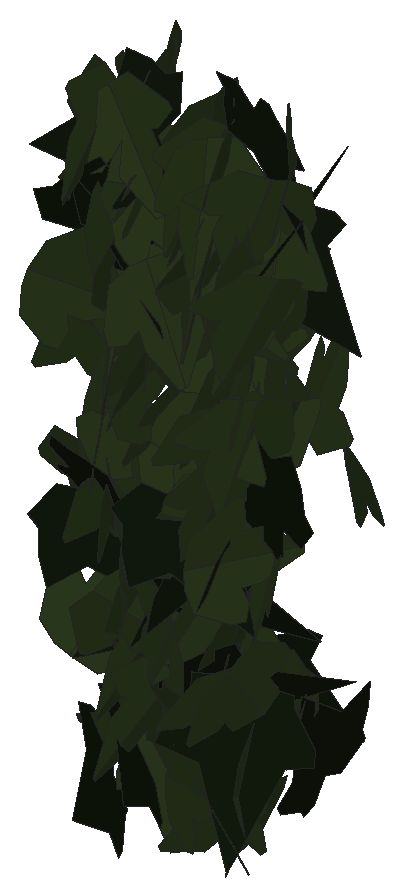
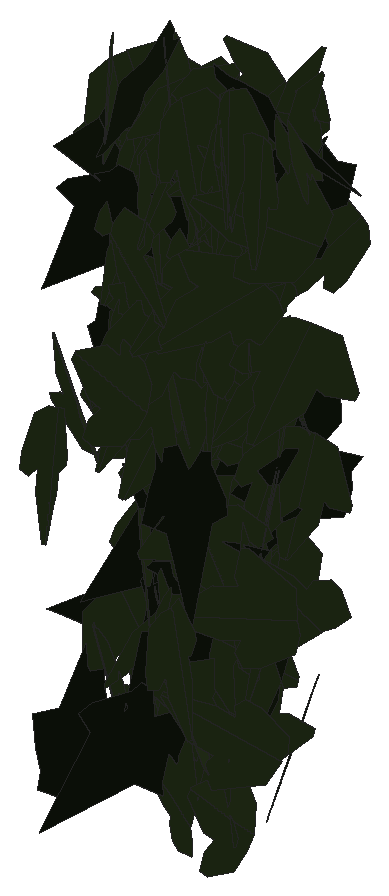
# SketchUp Ruby script. Lengths in inches.
U = 1.inch
M = Sketchup.active_model
def pt(a) = Geom::Point3d.new(a.map { |v| v * U })
def face(e, loops, mat)
  f = e.add_face(loops[0].map { |a| pt(a) })
  loops[1..].each { |l| e.add_face(l.map { |a| pt(a) }).erase! }
  f.material = f.back_material = mat if mat
  f
end
# faces: each face lists its corners as indices into pts; further lists are holes
def faces(e, pts, list, mat = nil) = list.each { |f| face(e, (f[0].is_a?(Array) ? f : [f]).map { |l| l.map { |i| pts[i] } }, mat) }
# xy, xz, yz: faces in a plane at the given z, y or x. An outline is a flat list of corners, or four numbers for a rectangle; further outlines are holes
def ring(l) = l.size == 4 ? [[l[0], l[1]], [l[2], l[1]], [l[2], l[3]], [l[0], l[3]]] : l.each_slice(2).to_a
def flat(e, list, mat, &to3) = list.each { |f| face(e, (f[0].is_a?(Array) ? f : [f]).map { |l| ring(l).map { |u, v| to3.(u, v) } }, mat) }
def xy(e, z, list, mat = nil) = flat(e, list, mat) { |x, y| [x, y, z] }
def xz(e, y, list, mat = nil) = flat(e, list, mat) { |x, z| [x, y, z] }
def yz(e, x, list, mat = nil) = flat(e, list, mat) { |y, z| [x, y, z] }
def lines(e, pts, list) = list.each { |a, b| e.add_line(pt(pts[a]), pt(pts[b])) }
# prism: a flat outline (further loops are holes) pulled along v
def prism(e, loops, v, mat = nil)
  f = face(e, loops, mat); d = Geom::Vector3d.new(v.map { |x| x * U })
  f.pushpull(f.normal.samedirection?(d) ? d.length : -d.length)
end
def box(e, o, s, mat = nil) = prism(e, [[o, [o[0] + s[0], o[1], o[2]], [o[0] + s[0], o[1] + s[1], o[2]], [o[0], o[1] + s[1], o[2]]]], [0, 0, s[2]], mat)
def at(x, y, z, deg = 0) = Geom::Transformation.translation(pt([x, y, z])) * Geom::Transformation.rotation(ORIGIN, Z_AXIS, deg.degrees)
def axes(o, x, y, z) = Geom::Transformation.new([*x, 0, *y, 0, *z, 0, *pt(o).to_a, 1])
def part(name) = M.definitions.add(name)
# library, detail: a bought-in or finely detailed component or shape, given as its bounding box
def library(name, o, s) = part(name).tap { |d| box(d.entities, o, s) }
def detail(e, o, s) = box(e.add_group.entities, o, s)
def put(e, d, t, mat = nil) = e.add_instance(d, t).tap { |i| i.material = mat if mat }
def group(e, t, mat = nil) = e.add_group.tap { |g| g.transformation = t; g.material = mat if mat }.entities
root = M.entities
M.materials.add("efeu1").color = [18, 25, 13]
M.materials.add("efeu2").color = [43, 57, 29]
c1 = part("ivyleaf_10")
p = [[0,0.5,-0.03],[-0.0625,2.02,-0.43],[-0.19,2.01,-0.46],[-0.54,1.05,-0.29],[-0.52,0.625,-0.18],[-0.83,0.76,-0.28],
  [-1.16,0.64,-0.33],[-1.15,0.33,-0.24],[-0.77,-0.39,0.02],[-0.3,-0.51,0.16],[0.04,-0.48,0.23],[-0.02,2.01,-0.4375],
  [-0.06,2.01,-0.43],[0.04,-0.49,0.23],[0.67,-0.49,0.14],[1.38,0.36,-0.2],[1.375,0.51,-0.24],[0.81,0.65,-0.19],
  [0.62,0.59,-0.15],[0.6,1.09,-0.28],[0.5,1.23,-0.31]]
faces(c1.entities,p,[[0,1,2,3,4,5,6,7,8,9,10],[11,12,0,13,14,15,16,17,18,19,20]],"efeu2")
c2 = part("ivyleaf_9")
p = [[1.54,2.16,1.25],[1.36,2.04,1.19],[-0.21,0.99,0.68],[-0.71,1.11,0.82],[-0.85,0.86,0.67],[-0.8,0.17,0.21],
  [-0.9,-0.01,0.1],[-0.67,-0.16,-0.02],[-0.08,-0.08,-0.05],[-0.03,-0.6,-0.4],[0.65,-0.88,-0.66],[0.83,-0.6,-0.49],
  [1.29,-0.42,-0.43],[1.8125,-0.07,-0.26],[1.21,0.44,0.15]]
faces(c2.entities,p,[[0,1,2,3,4,5,6,7,8,9,10,11,12,13,14]],"efeu1")
put(root,c1,axes([20.35,225.55,213.74],[-0.42421,0.23206,0.12727],[-0.13813,0.01099,-0.48042],[-0.22577,-0.44275,0.05478]))
put(root,c1,axes([20.23,225.05,211.57],[-0.33203,-0.30971,-0.20937],[0.1615,0.13372,-0.45391],[0.33715,-0.36905,0.01124]))
put(root,c1,axes([20.32,224.85,210.26],[-0.49854,0.03694,-0.0095],[0.00919,-0.0046,-0.49989],[-0.03702,-0.49861,0.00391]))
put(root,c1,axes([20.1875,225.09,213.93],[0.17199,-0.334,0.32994],[0.20812,-0.26073,-0.37243],[0.42084,0.26545,0.04934]))
put(root,c1,axes([19.99,225.76,209.06],[0.04249,-0.00209,0.49819],[0.40181,0.29574,-0.03303],[-0.29452,0.40316,0.02681]))
put(root,c1,axes([20.03,225.95,207.71],[0.24051,0.01866,-0.43796],[0.42744,0.10078,0.23903],[0.09719,-0.48938,0.03253]))
put(root,c1,axes([20.68,226.42,208.93],[-0.33019,0.13434,0.35061],[-0.33474,0.10614,-0.35592],[-0.17006,-0.46977,0.01985]))
put(root,c1,axes([20.4375,225.74,206.65],[0.14857,-0.34389,0.33116],[-0.11319,0.31157,0.37432],[-0.4638,-0.18619,0.01473]))
put(root,c1,axes([20.18,225.2,212.86],[-0.04588,-0.26731,0.42005],[0.27754,0.33648,0.24444],[-0.41336,0.25559,0.11751]))
put(root,c1,axes([20.53,225.05,208.63],[-0.22189,0.36487,0.26007],[-0.12953,0.22558,-0.42701],[-0.42894,-0.25687,-0.00559]))
put(root,c1,axes([20.53,225.11,211.0625],[-0.0182,0.02508,0.49904],[-0.16563,0.47084,-0.0297],[-0.47142,-0.16639,-0.00883]))
put(root,c1,axes([20.39,224.25,212.4],[0.08449,0.23876,0.43111],[0.03337,0.43362,-0.24669],[-0.49168,0.07045,0.05734]))
put(root,c1,axes([20.34,224.81,208.51],[0.37458,0.16086,-0.28951],[0.24278,0.16391,0.4052],[0.22526,-0.44414,0.04469]))
put(root,c2,axes([20.41,225.08,206.9],[-0.00427,-0.18194,0.4657],[-0.00756,-0.46564,-0.18199],[0.49992,-0.0086,0.00122]))
put(root,c1,axes([20.45,224.9,213.9375],[0.03692,-0.24307,0.43538],[0.20982,-0.38847,-0.23467],[0.45234,0.20003,0.07332]))
put(root,c1,axes([20.62,225.56,214.13],[0.10374,-0.45853,-0.17026],[0.0077,0.17555,-0.4681],[0.48906,0.0945,0.04349]))
put(root,c1,axes([20.6,224.87,210.22],[-0.09866,-0.40844,-0.271],[0.08151,0.25892,-0.4199],[0.48334,-0.12703,0.0155]))
put(root,c2,axes([20.47,224.69,210],[0.05034,-0.28739,-0.40604],[-0.0587,0.40183,-0.29169],[0.49398,0.07703,0.00672]))
put(root,c2,axes([21.04,224.89,213.85],[-0.39263,0.17549,0.25504],[-0.23259,0.10463,-0.43006],[-0.20431,-0.45635,-0.00053]))
put(root,c1,axes([20.55,224.81,211.17],[0.31965,-0.31389,0.22203],[0.16947,-0.14415,-0.44777],[0.34511,0.36152,0.01423]))
put(root,c1,axes([20.8125,225.66,206.73],[0.41253,-0.1131,0.2589],[-0.25032,0.06611,0.42775],[-0.13099,-0.48253,-0.00207]))
put(root,c1,axes([20.72,225.52,214.04],[0.2006,-0.44315,-0.11565],[-0.00035,0.12611,-0.48383],[0.45799,0.1942,0.05028]))
put(root,c1,axes([20.79,225.19,207.3],[-0.49327,-0.06669,-0.04734],[-0.04611,-0.01224,0.49772],[-0.06755,0.49538,0.00593]))
put(root,c2,axes([20.86,225.93,210.35],[0.29065,0.05672,-0.40287],[-0.40003,-0.05043,-0.29569],[-0.07418,0.49421,0.01607]))
put(root,c1,axes([20.78,224.57,210.31],[0.18456,-0.30964,-0.3465],[-0.03849,0.36136,-0.34342],[0.46309,0.15343,0.10955]))
put(root,c1,axes([21.03,224.83,211.83],[-0.38527,-0.00181,0.31869],[-0.31868,0.00717,-0.38522],[-0.00317,-0.49995,-0.00668]))
put(root,c1,axes([20.76,225.41,211.69],[-0.12886,-0.28149,0.39263],[0.08962,-0.41323,-0.26685],[0.47473,0.00161,0.15695]))
put(root,c2,axes([20.4,224.59,210.26],[0.42293,-0.17193,0.2039],[0.18841,-0.07796,-0.45653],[0.18877,0.46299,-0.00116]))
put(root,c1,axes([20.65,225.09,208.6875],[0.31954,-0.37028,-0.10385],[0.06589,-0.08032,0.48909],[-0.37888,-0.32626,-0.00253]))
put(root,c1,axes([20.83,224.77,210.58],[0.02375,0.4817,-0.1319],[-0.00289,0.13218,0.4822],[0.49943,-0.02215,0.00907]))
put(root,c2,axes([20.5,224.84,213.05],[0.28042,-0.40259,0.09636],[0.05111,-0.08182,-0.4906],[0.41079,0.285,-0.00473]))
put(root,c2,axes([20.42,224.65,212.79],[0.1692,0.01649,0.47021],[0.46785,0.04707,-0.17],[-0.04987,0.49751,0.0005]))
put(root,c1,axes([20.52,225.52,212.25],[0.21402,0.18153,0.41381],[0.26213,0.32309,-0.2773],[-0.36808,0.33565,0.04313]))
put(root,c1,axes([20.57,225.1,209.3125],[0.03419,-0.08632,0.4913],[0.37292,-0.32265,-0.08264],[0.3313,0.37209,0.04232]))
put(root,c1,axes([20.79,224.6875,210.25],[-0.20306,-0.37306,-0.2638],[0.14297,0.2223,-0.42443],[0.43396,-0.2478,0.01639]))
put(root,c1,axes([20.86,225.7,209.69],[0.39943,0.2764,-0.11856],[-0.09335,-0.07344,-0.48569],[-0.2859,0.41014,-0.00707]))
put(root,c1,axes([20.76,225.11,208.45],[0.02032,-0.14872,0.47694],[0.20688,-0.43198,-0.14352],[0.45474,0.20317,0.04398]))
put(root,c1,axes([20.82,225.85,207.86],[0.23116,-0.38342,0.22261],[0.09801,-0.20065,-0.44736],[0.43239,0.25046,-0.01761]))
put(root,c1,axes([20.97,224.1875,212.86],[0.0093,0.03412,-0.49875],[-0.05156,0.49624,0.03298],[0.49725,0.05082,0.01275]))
put(root,c2,axes([21.2,225.51,209.125],[-0.43767,-0.17221,0.16968],[-0.1582,-0.06135,-0.47033],[0.18281,-0.46538,-0.00079]))
put(root,c2,axes([20.75,225.03,207.33],[0.01301,-0.23055,0.44348],[0.08072,-0.43684,-0.22947],[0.49327,0.07757,0.02585]))
put(root,c1,axes([20.64,226.25,206.96],[-0.06938,-0.00166,0.49516],[0.47617,-0.13736,0.06626],[0.13581,0.48076,0.02064]))
put(root,c1,axes([20.8125,224.64,209.05],[-0.3066,-0.16633,-0.35823],[0.30662,0.18561,-0.34861],[0.24896,-0.43345,-0.01181]))
put(root,c1,axes([20.91,225.4,207.28],[0.31898,0.38503,-0.00009],[-0.00391,0.00312,-0.49997],[-0.38501,0.31897,0.005]))
put(root,c1,axes([21.03,225.03,208.06],[0.01427,-0.30623,0.39499],[0.03793,-0.39335,-0.30633],[0.49836,0.0387,0.012]))
put(root,c1,axes([20.93,224.88,208.84],[-0.01111,-0.42401,0.26475],[0.04726,0.26274,0.42277],[-0.49764,0.03442,0.03424]))
put(root,c1,axes([21.0625,225.0625,213.43],[0.02805,-0.45958,-0.19494],[0.02291,0.19622,-0.45932],[0.49869,0.01684,0.03206]))
put(root,c1,axes([20.74,224.73,214.05],[0.3627,0.04762,0.34085],[0.3404,0.02337,-0.36549],[-0.05074,0.49718,-0.01547]))
put(root,c1,axes([21.1875,224.33,211.49],[-0.01977,0.04872,0.49723],[-0.19779,0.4562,-0.05256],[-0.45879,-0.19877,0.00124]))
put(root,c1,axes([21.1875,224.57,211.74],[0.10338,-0.43156,-0.23036],[-0.06496,0.22125,-0.44365],[0.48486,0.12165,-0.01032]))
put(root,c1,axes([20.92,224.71,213.4],[-0.05814,-0.19727,-0.45575],[0.32626,0.33077,-0.18479],[0.3744,-0.31887,0.09026]))
put(root,c1,axes([21.16,225.37,209.58],[-0.11444,-0.3912,0.2896],[0.04,-0.30405,-0.39491],[0.48508,-0.06722,0.10088]))
put(root,c1,axes([21.18,225.53,213.85],[-0.01947,-0.49945,-0.01301],[-0.00142,0.01308,-0.49983],[0.49962,-0.01943,-0.00193]))
put(root,c1,axes([21.13,224.99,213.47],[-0.15831,-0.41361,-0.23209],[0.10317,0.20878,-0.44245],[0.46292,-0.18798,0.01924]))
put(root,c1,axes([21.2,224.92,211.17],[-0.01052,-0.43562,-0.2452],[0.00108,0.24523,-0.43573],[0.49989,-0.0097,-0.00422]))
put(root,c1,axes([21.1,225.39,212.14],[-0.0826,-0.21026,-0.44606],[0.16002,0.41637,-0.2259],[0.46644,-0.18008,-0.0015]))
put(root,c1,axes([21.16,224.89,208.9],[-0.27202,0.36763,0.20212],[0.09832,-0.17832,0.45666],[0.40785,0.28818,0.02472]))
put(root,c2,axes([21.15,226.15,207.71],[0.02051,-0.082,-0.4928],[-0.06213,0.48897,-0.08395],[0.4957,0.06468,0.00987]))
put(root,c1,axes([21.27,225.37,213.35],[0.49757,0.04734,-0.01367],[-0.01411,0.00403,-0.49978],[-0.04721,0.49774,0.00534]))
put(root,c1,axes([21.41,225.52,210.97],[-0.18903,-0.46234,0.02259],[-0.00831,-0.02101,-0.49949],[0.46282,-0.18921,0.00026]))
put(root,c1,axes([21.68,224.47,208.49],[-0.11041,0.04006,0.48601],[-0.46529,0.14054,-0.11729],[-0.14601,-0.47817,0.00625]))
put(root,c1,axes([21.4,225.13,213.24],[0.16198,-0.45062,-0.14387],[-0.02766,0.14279,-0.47838],[0.47223,0.16293,0.02133]))
put(root,c1,axes([21.33,226.26,211.15],[0.11795,-0.38713,0.29363],[-0.05065,0.29071,0.40363],[-0.48324,-0.12496,0.02936]))
put(root,c1,axes([21.37,224.77,212.31],[-0.20364,-0.39787,-0.22412],[0.0867,0.20725,-0.44669],[0.44835,-0.22079,-0.01542]))
put(root,c1,axes([21.05,224.67,213.31],[0.23246,0.13764,0.42074],[0.33455,0.25658,-0.26878],[-0.28989,0.40648,0.02719]))
put(root,c1,axes([21.37,225.71,211.65],[-0.22274,-0.3644,-0.26],[0.15269,0.21115,-0.42673],[0.4208,-0.2695,0.01722]))
put(root,c1,axes([21.48,225.27,210.98],[0.17113,-0.4698,-0.00196],[-0.00068,0.00184,-0.5],[0.4698,0.17113,-0.00001]))
put(root,c1,axes([21.49,225.2,209.09],[0.05469,0.25198,-0.42838],[-0.09321,-0.41812,-0.25785],[-0.48818,0.10807,0.00124]))
put(root,c2,axes([21.65,225.09,208.375],[-0.08006,0.09682,-0.48396],[-0.34159,0.34302,0.12513],[0.35624,0.35067,0.01122]))
put(root,c1,axes([21.38,224.49,212.5625],[0.27901,0.39145,0.13754],[0.06249,0.12421,-0.48028],[-0.41018,0.28519,0.02039]))
put(root,c1,axes([21.5,225.15,213.73],[-0.02195,-0.39493,0.30586],[0.08769,-0.30445,-0.38681],[0.49176,0.03666,0.08262]))
put(root,c1,axes([21.8,225.7,212.36],[0.13292,-0.09129,-0.47328],[-0.34937,0.31999,-0.15984],[0.33207,0.3732,0.02128]))
put(root,c1,axes([21.59,225.29,206.81],[-0.21379,-0.39157,-0.22575],[-0.09962,-0.20277,0.44605],[-0.44087,0.2357,0.00869]))
put(root,c1,axes([21.57,225.11,213.21],[0.03889,-0.29915,-0.39874],[0.0481,0.40034,-0.29566],[0.49616,-0.01536,0.05991]))
put(root,c1,axes([21.56,225.6,208.36],[-0.01631,0.47485,-0.15573],[0.01007,-0.15547,-0.47511],[-0.49963,-0.01863,-0.00449]))
put(root,c1,axes([21.73,224.46,207.56],[-0.10289,0.28168,0.40009],[-0.18525,0.35598,-0.29826],[-0.45287,-0.20961,0.03111]))
put(root,c1,axes([21.56,224.93,212.62],[0.00893,-0.12676,-0.48358],[0.02166,-0.48311,0.12703],[-0.49945,-0.02322,-0.00314]))
put(root,c2,axes([21.83,224.78,210.03],[-0.43841,0.2005,-0.13266],[0.12138,-0.05357,-0.48208],[-0.20752,-0.4549,-0.0017]))
put(root,c1,axes([21.33,224.84,210.31],[0.22201,0.05533,-0.44458],[0.43529,0.09075,0.22867],[0.106,-0.48857,-0.00787]))
put(root,c2,axes([21.44,224.93,209.35],[0.44351,0.1804,0.14406],[0.1318,0.05831,-0.47878],[-0.18955,0.46266,0.00416]))
put(root,c1,axes([21.77,225.23,213],[0.0593,-0.46712,-0.16818],[-0.03486,0.16504,-0.47069],[0.49525,0.06755,-0.01299]))
put(root,c2,axes([21.5,224.62,210.33],[0.11002,-0.38084,-0.30473],[0.00649,0.3135,-0.38946],[0.4877,0.08175,0.07393]))
put(root,c1,axes([21.9375,225.49,208.33],[-0.36569,-0.22872,0.25289],[-0.20897,-0.1427,-0.43124],[0.26944,-0.4211,0.00877]))
put(root,c1,axes([21.79,225.39,209.15],[0.17833,-0.41666,-0.21117],[-0.06427,0.202,-0.45284],[0.46267,0.18865,0.01849]))
put(root,c1,axes([21.69,224.86,213.75],[0.17322,0.45611,-0.10938],[-0.05178,-0.09729,-0.4877],[-0.46617,0.18028,0.01353]))
put(root,c1,axes([21.8,225.01,214.05],[0.2077,-0.42499,-0.162],[-0.03569,0.16231,-0.47157],[0.45341,0.20746,0.03709]))
put(root,c1,axes([21.57,224.67,210.19],[-0.16498,-0.16742,-0.44131],[0.3006,0.32315,-0.23497],[0.3639,-0.34284,-0.00598]))
put(root,c1,axes([21.53,225.39,211.68],[0.3506,0.26188,0.24186],[0.20154,0.1342,-0.43746],[-0.29404,0.40424,-0.01146]))
put(root,c1,axes([21.73,225.05,210.47],[-0.19315,-0.35434,-0.29519],[0.13407,0.26307,-0.40351],[0.44127,-0.23502,-0.00661]))
put(root,c1,axes([21.77,224.86,211.09],[0.49466,0.02384,-0.06887],[-0.06876,-0.00376,-0.49523],[-0.02413,0.49942,-0.00044]))
put(root,c1,axes([21.83,225.18,209.1],[0.12,-0.48073,-0.06709],[-0.01181,0.0662,-0.49546],[0.48524,0.1205,0.00454]))
put(root,c1,axes([21.5,224.9,212.36],[-0.26891,-0.01567,-0.42124],[0.42029,0.02837,-0.26935],[0.03234,-0.49895,-0.00209]))
put(root,c1,axes([21.77,225.54,211.02],[0.00856,-0.40829,-0.28849],[0.09876,0.28423,-0.39933],[0.49007,-0.05015,0.08551]))
put(root,c1,axes([21.84,225.05,211.73],[-0.01632,-0.4424,-0.23242],[0.01383,0.23205,-0.44267],[0.49954,-0.02088,0.00467]))
put(root,c1,axes([21.85,225.43,210.61],[0.21567,0.44612,0.06678],[-0.03332,-0.05806,0.4955],[0.44986,-0.21818,0.00468]))
put(root,c1,axes([21.7,224.83,212.9],[0.31032,-0.32331,0.22175],[0.14481,-0.16828,-0.44801],[0.36432,0.34227,-0.0108]))
put(root,c1,axes([21.89,224.84,210.64],[0.0153,-0.46887,0.173],[0.01113,-0.17272,-0.46909],[0.49964,0.01821,0.00515]))
put(root,c2,axes([21.52,224.89,208.21],[0.28358,0.04152,0.40971],[0.38491,0.15011,-0.28163],[-0.14638,0.47513,0.05317]))
put(root,c2,axes([21.5,224.98,207.21],[0.31687,-0.0627,-0.38165],[0.37261,-0.08278,0.32297],[-0.10369,-0.4891,-0.00574]))
put(root,c1,axes([21.97,224.96,211.66],[0.32415,-0.34227,-0.16667],[-0.10581,0.12928,-0.47127],[0.36569,0.34079,0.01138]))
put(root,c1,axes([22,225.75,208],[0.32698,-0.35411,-0.13301],[-0.08404,0.10341,-0.48192],[0.36881,0.33751,0.00811]))
put(root,c1,axes([21.96,224.73,211.26],[-0.30185,-0.37591,-0.13258],[0.09414,0.09436,-0.48191],[0.38733,-0.31589,0.01381]))
put(root,c1,axes([21.82,226.31,210.66],[0.39196,-0.27961,-0.13486],[0.11076,-0.07695,0.48147],[-0.29,-0.4073,0.00162]))
put(root,c1,axes([21.99,225.18,212.58],[-0.11678,-0.41471,-0.25373],[0.1146,0.23011,-0.42885],[0.47247,-0.15831,0.04131]))
put(root,c2,axes([21.73,225.53,214.02],[0.24027,-0.41062,0.15383],[0.07852,-0.13228,-0.47575],[0.4314,0.25277,0.00092]))
put(root,c2,axes([21.96,226.24,206.98],[0.12,0.23287,0.42588],[-0.1916,-0.38035,0.26197],[0.44597,-0.22607,-0.00205]))
put(root,c2,axes([21.8,225.51,212.83],[-0.05749,-0.20645,-0.45174],[0.18141,0.41461,-0.21257],[0.46237,-0.18835,0.02723]))
put(root,c1,axes([22.1,225.25,211.33],[0.04482,-0.25111,-0.43004],[-0.00338,0.43161,-0.25239],[0.49798,0.02553,0.037]))
put(root,c1,axes([22.13,224.58,208.66],[-0.14063,-0.4785,-0.03552],[0.00619,0.0352,-0.49872],[0.47978,-0.14071,-0.00398]))
put(root,c1,axes([22.08,224.85,212.99],[0.05094,-0.37495,-0.32683],[0.07325,0.33062,-0.36787],[0.49197,-0.01041,0.08861]))
put(root,c1,axes([22.16,224.9,211.26],[-0.19037,-0.44096,0.13898],[0.00137,-0.15084,-0.4767],[0.46234,-0.18111,0.05864]))
put(root,c1,axes([22.16,224.86,213.05],[-0.00707,-0.41918,-0.27246],[0.06334,0.26955,-0.41633],[0.49592,-0.0404,0.04929]))
put(root,c1,axes([22.33,226.17,210.4],[-0.38743,0.22976,0.21704],[-0.19091,0.10351,-0.45038],[-0.25189,-0.43185,0.00752]))
put(root,c1,axes([22.1,224.42,209.93],[0.00181,0.03289,0.49891],[0.02867,0.49809,-0.03294],[-0.49917,0.02873,-0.00009]))
put(root,c1,axes([22.35,224.87,213.67],[-0.31736,-0.35415,0.15446],[-0.09475,-0.12244,-0.47543],[0.37457,-0.33103,0.0106]))
put(root,c1,axes([22.4,224.56,207.625],[-0.10311,0.11983,0.47435],[-0.29646,0.37033,-0.158],[-0.3892,-0.31383,-0.00531]))
put(root,c2,axes([22.25,224.95,212.83],[-0.23138,0.40523,-0.17959],[-0.09028,0.15525,0.46663],[0.43395,0.24836,0.00132]))
put(root,c1,axes([22.13,224.89,206.97],[0.14046,-0.4773,-0.04952],[0.02692,-0.04368,0.49736],[-0.47911,-0.14238,0.01343]))
put(root,c1,axes([22.375,225.16,213.84],[0.08666,-0.22004,-0.44054],[-0.14546,0.41591,-0.23635],[0.47046,0.16913,0.00807]))
put(root,c1,axes([22.24,225.125,212.48],[-0.04171,-0.33645,0.36751],[0.05433,-0.36967,-0.33226],[0.49529,0.01221,0.06739]))
put(root,c1,axes([22.25,225.06,209.82],[0.36984,-0.33486,0.03288],[0.02743,-0.01869,-0.4989],[0.33535,0.37083,0.00455]))
put(root,c2,axes([22.21,224.82,208.3],[-0.18837,-0.45511,-0.08597],[0.03844,0.07713,-0.49252],[0.46156,-0.19217,0.00593]))
put(root,c1,axes([22.28,224.56,208.75],[-0.14689,-0.38055,-0.28915],[0.09924,0.27162,-0.40789],[0.46752,-0.17722,-0.00427]))
put(root,c2,axes([22.58,224.82,210.39],[0.06994,-0.11497,0.48155],[-0.27968,0.39212,0.13423],[-0.40852,-0.28814,-0.00946]))
put(root,c1,axes([22.48,224.73,212.73],[-0.18305,-0.42472,0.19001],[-0.07725,-0.17361,-0.46249],[0.45883,-0.19867,-0.00206]))
put(root,c1,axes([22.27,225.12,213.07],[0.499,-0.00809,0.03063],[0.03066,0.00182,-0.49906],[0.00797,0.49993,0.00232]))
